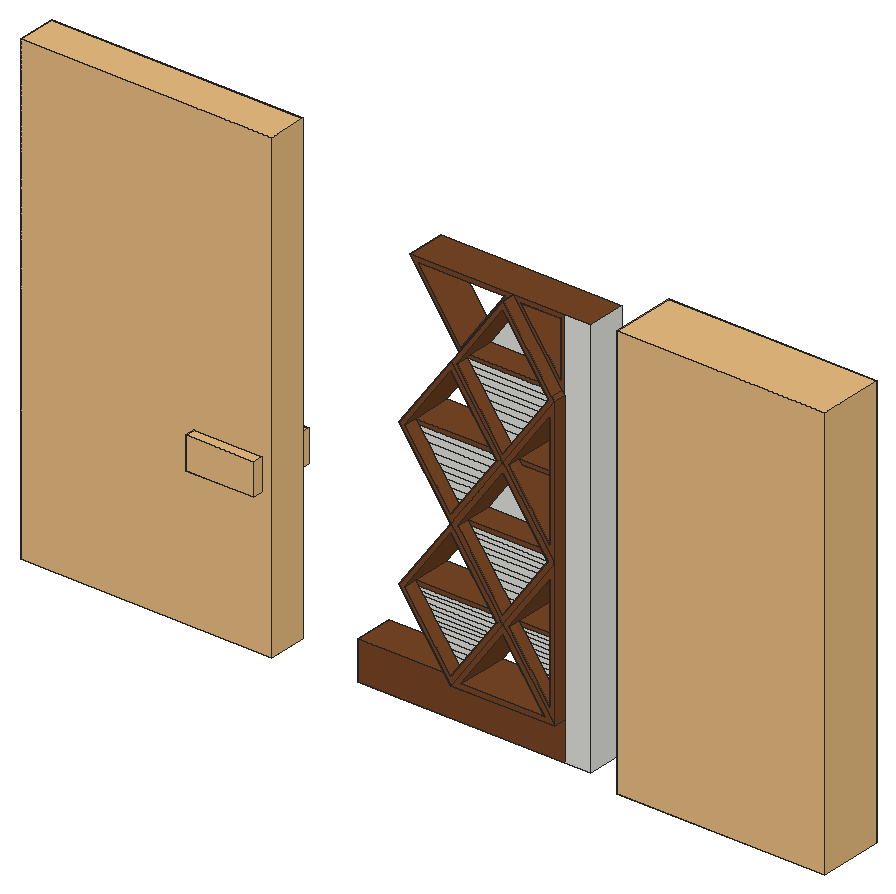
# SketchUp Ruby script. Lengths in inches.
U = 1.inch
M = Sketchup.active_model
def pt(a) = Geom::Point3d.new(a.map { |v| v * U })
def face(e, loops, mat)
  f = e.add_face(loops[0].map { |a| pt(a) })
  loops[1..].each { |l| e.add_face(l.map { |a| pt(a) }).erase! }
  f.material = f.back_material = mat if mat
  f
end
# faces: each face lists its corners as indices into pts; further lists are holes
def faces(e, pts, list, mat = nil) = list.each { |f| face(e, (f[0].is_a?(Array) ? f : [f]).map { |l| l.map { |i| pts[i] } }, mat) }
# xy, xz, yz: faces in a plane at the given z, y or x. An outline is a flat list of corners, or four numbers for a rectangle; further outlines are holes
def ring(l) = l.size == 4 ? [[l[0], l[1]], [l[2], l[1]], [l[2], l[3]], [l[0], l[3]]] : l.each_slice(2).to_a
def flat(e, list, mat, &to3) = list.each { |f| face(e, (f[0].is_a?(Array) ? f : [f]).map { |l| ring(l).map { |u, v| to3.(u, v) } }, mat) }
def xy(e, z, list, mat = nil) = flat(e, list, mat) { |x, y| [x, y, z] }
def xz(e, y, list, mat = nil) = flat(e, list, mat) { |x, z| [x, y, z] }
def yz(e, x, list, mat = nil) = flat(e, list, mat) { |y, z| [x, y, z] }
def lines(e, pts, list) = list.each { |a, b| e.add_line(pt(pts[a]), pt(pts[b])) }
# prism: a flat outline (further loops are holes) pulled along v
def prism(e, loops, v, mat = nil)
  f = face(e, loops, mat); d = Geom::Vector3d.new(v.map { |x| x * U })
  f.pushpull(f.normal.samedirection?(d) ? d.length : -d.length)
end
def box(e, o, s, mat = nil) = prism(e, [[o, [o[0] + s[0], o[1], o[2]], [o[0] + s[0], o[1] + s[1], o[2]], [o[0], o[1] + s[1], o[2]]]], [0, 0, s[2]], mat)
def at(x, y, z, deg = 0) = Geom::Transformation.translation(pt([x, y, z])) * Geom::Transformation.rotation(ORIGIN, Z_AXIS, deg.degrees)
def axes(o, x, y, z) = Geom::Transformation.new([*x, 0, *y, 0, *z, 0, *pt(o).to_a, 1])
def part(name) = M.definitions.add(name)
# library, detail: a bought-in or finely detailed component or shape, given as its bounding box
def library(name, o, s) = part(name).tap { |d| box(d.entities, o, s) }
def detail(e, o, s) = box(e.add_group.entities, o, s)
def put(e, d, t, mat = nil) = e.add_instance(d, t).tap { |i| i.material = mat if mat }
def group(e, t, mat = nil) = e.add_group.tap { |g| g.transformation = t; g.material = mat if mat }.entities
root = M.entities
M.materials.add("[Wood Veneer 01]").color = [120, 70, 37]
c1 = library("Group4\#1",[-223.39,66.61,0],[17.37,17.18,34.03])
c2 = library("Group145\#1",[5.875,6.46,9.56],[20.8,10.13,11.36])
c3 = library("Redhome_Model_Tree_04",[-24.25,-16.26,0],[46.77,28.59,38.54])
c4 = library("Deer Decoration @ADS 031224",[-97.53,29.72,25.79],[8.17,5.75,13.32])
c5 = library("MC-5",[1.46,3.91,28.72],[9.58,10.53,13.64])
c6 = library("DECOR4",[0,0,0],[6.14,2.35,8.66])
c7 = library("Vaso+com+Suculentas+e+Livro+Chanel+-+Marilia+Zimmermann",[189.86,96.28,0],[20.19,20.19,9.48])
c8 = library("Decor 1 - asm",[600.96,98.01,0],[8.71,8.72,11.09])
c9 = library("Group\#1",[0,0,0],[19.39,3,36])
c10 = library("Group43\#1",[-4.22,-4.32,0],[4.42,4.42,11.16])
c11 = library("Group43",[-4.22,-4.32,0],[4.42,4.42,11.16])
c12 = library("Group\#127",[-0.03,-0.72,0],[16.04,5,32])
xy(root,0,[[0,1,18,4]])
xy(root,2.96,[[8,0,16,1],[0,1,8,4]],"[Wood Veneer 01]")
xy(root,3.35,[[8.77,0,15.23,4]],"[Wood Veneer 01]")
xy(root,8.5625,[[4.47,1,11.53,4],[12.47,1,15.62,4]],"[Wood Veneer 01]")
xy(root,14.17,[[8.5,1,15.5,3]],"[Wood Veneer 01]")
xy(root,19.47,[[12.68,1,15.625,3]],"[Wood Veneer 01]")
xy(root,19.77,[[4.47,1,11.53,4],[12.46,1,15.625,4]],"[Wood Veneer 01]")
xy(root,25.66,[[8.66,1,15.34,3]],"[Wood Veneer 01]")
xy(root,30.66,[[4.62,1,11.38,4],[12.62,1,15.68,4]],"[Wood Veneer 01]")
xy(root,30.98,[[4,1,18,4]],"[Wood Veneer 01]")
xz(root,0,[[8,2.96,11.8,8.28,12,8.5625,11.53,8.5625,11.33,8.28,8,3.62,4.47,8.5625,8,13.5,11.53,8.5625,12,8.5625,8.24,13.83,8,14.17,4,8.5625],[[8,2.96,16,2.96,12.21,8.26,12,8.5625,11.8,8.28],[8.77,3.35,12,7.88,15.23,3.35]],[[16,2.96,16,14.17,15.76,13.83,12,8.5625,12.21,8.26],[15.62,4.14,12.68,8.26,12.47,8.5625,15.62,12.98]],[[12,8.5625,15.76,13.83,16,14.17,12,19.77,11.74,19.41,8,14.17,8.24,13.83],[12,9.26,8.74,13.83,8.5,14.17,12,19.07,15.5,14.17,15.26,13.83]],[8,14.17,11.74,19.41,12,19.77,11.53,19.77,11.27,19.41,8,14.83,4.47,19.77,8,24.72,11.53,19.77,12,19.77,8,25.375,4,19.77],
  [[16,14.17,16,25.375,12,19.77],[15.625,15.34,12.68,19.47,12.46,19.77,15.625,24.2]],[[12,19.77,16,25.375,15.8,25.66,12,30.98,8.2,25.66,8,25.375],[12,20.42,8.46,25.375,8.66,25.66,12,30.33,15.34,25.66,15.54,25.375]]],"[Wood Veneer 01]")
xz(root,1,[[16,0,18,30.98],[8,3.62,8.53,4.37,7.47,4.37],[15.62,4.14,15.62,4.99,15.02,4.99],[7.47,4.37,8.53,4.37,8.82,4.77,7.18,4.77],[7.18,4.77,8.82,4.77,9.125,5.2,6.875,5.2],
  [15.02,4.99,15.62,4.99,15.62,5.3125,14.79,5.3125],[6.875,5.2,9.125,5.2,9.45,5.65,6.55,5.65],[14.79,5.3125,15.62,5.3125,15.62,5.625,14.5625,5.625],[14.5625,5.625,15.62,5.625,15.62,5.98,14.31,5.98],[6.55,5.65,9.45,5.65,9.72,6.02,6.28,6.02],
  [14.31,5.98,15.62,5.98,15.62,6.32,14.07,6.32],[6.28,6.02,9.72,6.02,9.94,6.34,6.06,6.34],[14.07,6.32,15.62,6.32,15.62,6.68,13.81,6.68],[6.06,6.34,9.94,6.34,10.18,6.68,5.82,6.68],[5.82,6.68,10.18,6.68,10.39,6.96,5.61,6.96],
  [13.81,6.68,15.62,6.68,15.62,7.02,13.57,7.02],[5.61,6.96,10.39,6.96,10.64,7.32,5.36,7.32],[13.57,7.02,15.62,7.02,15.62,7.34,13.34,7.34],[5.36,7.32,10.64,7.32,10.9,7.68,5.1,7.68],[13.34,7.34,15.62,7.34,15.62,7.68,13.1,7.68],
  [5.1,7.68,10.9,7.68,11.125,8,4.875,8],[13.1,7.68,15.62,7.68,15.62,8.02,12.85,8.02],[4.875,8,11.125,8,11.33,8.28,4.67,8.28],[12.85,8.02,15.62,8.02,15.62,8.26,12.68,8.26],[12,9.26,12.42,9.84,11.58,9.84],
  [11.58,9.84,12.42,9.84,12.83,10.42,11.17,10.42],[11.17,10.42,12.83,10.42,13.18,10.92,10.82,10.92],[10.82,10.92,13.18,10.92,13.56,11.44,10.44,11.44],[10.44,11.44,13.56,11.44,13.85,11.85,10.15,11.85],[10.15,11.85,13.85,11.85,14.1875,12.32,9.8125,12.32],
  [9.8125,12.32,14.1875,12.32,14.48,12.74,9.52,12.74],[9.52,12.74,14.48,12.74,14.77,13.14,9.23,13.14],[9.23,13.14,14.77,13.14,15.03,13.5,8.97,13.5],[8.97,13.5,15.03,13.5,15.26,13.83,8.74,13.83],[8,14.83,8.4,15.38,7.6,15.38],
  [7.6,15.38,8.4,15.38,8.79,15.9375,7.21,15.9375],[7.21,15.9375,8.79,15.9375,9.16,16.45,6.84,16.45],[6.84,16.45,9.16,16.45,9.4375,16.84,6.5625,16.84],[6.5625,16.84,9.4375,16.84,9.79,17.33,6.21,17.33],[6.21,17.33,9.79,17.33,10.18,17.88,5.82,17.88],
  [5.82,17.88,10.18,17.88,10.58,18.45,5.42,18.45],[5.42,18.45,10.58,18.45,10.98,19,5.02,19],[5.02,19,10.98,19,11.27,19.41,4.73,19.41],[12,20.42,12.67,21.36,11.33,21.36],[11.33,21.36,12.67,21.36,13.09,21.9375,10.91,21.9375],
  [10.91,21.9375,13.09,21.9375,13.5,22.52,10.5,22.52],[10.5,22.52,13.5,22.52,13.875,23.04,10.125,23.04],[10.125,23.04,13.875,23.04,14.25,23.58,9.75,23.58],[9.75,23.58,14.25,23.58,14.54,23.98,9.46,23.98],[9.46,23.98,14.54,23.98,14.89,24.47,9.11,24.47],
  [9.11,24.47,14.89,24.47,15.21,24.91,8.79,24.91],[8.79,24.91,15.21,24.91,15.54,25.375,8.46,25.375]])
xz(root,1,[[0,0,16,2.96],[12.68,8.26,15.62,8.26,15.62,8.5625,12.47,8.5625],[4.67,8.28,11.33,8.28,11.53,8.5625,4.47,8.5625],[8.74,13.83,15.26,13.83,15.5,14.17,8.5,14.17],[4.73,19.41,11.27,19.41,11.53,19.77,4.47,19.77],
  [12.68,19.47,15.625,19.47,15.625,19.77,12.46,19.77],[[8,25.375,8.2,25.66,12,30.98,15.8,25.66,16,25.375,16,30.98,4,30.98],[8,25.92,4.62,30.66,11.38,30.66],[15.68,26.37,12.62,30.66,15.68,30.66]],[8.46,25.375,15.54,25.375,15.34,25.66,8.66,25.66]],"[Wood Veneer 01]")
xz(root,3,[[8.5,14.17,15.5,14.17,12,19.07],[8.66,25.66,15.34,25.66,12,30.33]])
xz(root,3.97,[[11.9,8.41,7.9,14.02,8,14.17,11.9,19.62,15.9,14.02]])
yz(root,0,[[1,0,4,2.96]],"[Wood Veneer 01]")
yz(root,15.62,[[0,4.14,0,12.98,4,12.98,4,8.5625,1,8.5625,1,4.14]],"[Wood Veneer 01]")
yz(root,15.625,[[0,15.34,3,19.47],[0,19.47,1,19.77],[0,19.77,4,24.2]],"[Wood Veneer 01]")
yz(root,15.68,[[1,26.37,4,30.66]],"[Wood Veneer 01]")
yz(root,16,[[0,2.96,1,25.375]],"[Wood Veneer 01]")
yz(root,18,[[1,0,4,30.98]])
p = [[4,0,8.5625],[4,4,8.5625],[8,4,2.96],[8,1,2.96],[8,0,2.96],[12,4,7.88],
  [12,0,7.88],[8.77,0,3.35],[8.77,4,3.35],[15.23,4,3.35],[15.23,0,3.35],[4.875,1,8],
  [4.67,1,8.28],[4.47,1,8.5625],[4.47,0,8.5625],[8,0,3.62],[8,1,3.62],[7.47,1,4.37],
  [7.18,1,4.77],[6.875,1,5.2],[6.55,1,5.65],[6.28,1,6.02],[6.06,1,6.34],[5.82,1,6.68],
  [5.61,1,6.96],[5.36,1,7.32],[5.1,1,7.68],[11.53,1,8.5625],[11.33,1,8.28],[11.125,1,8],
  [10.9,1,7.68],[10.64,1,7.32],[10.39,1,6.96],[10.18,1,6.68],[9.94,1,6.34],[9.72,1,6.02],
  [9.45,1,5.65],[9.125,1,5.2],[8.82,1,4.77],[8.53,1,4.37],[11.33,0,8.28],[11.53,0,8.5625],
  [12.85,1,8.02],[12.68,1,8.26],[12.47,1,8.5625],[12.47,0,8.5625],[12.68,0,8.26],[15.62,0,4.14],
  [15.62,1,4.14],[15.02,1,4.99],[14.79,1,5.3125],[14.5625,1,5.625],[14.31,1,5.98],[14.07,1,6.32],
  [13.81,1,6.68],[13.57,1,7.02],[13.34,1,7.34],[13.1,1,7.68],[11.9,1.97,8.41],[7.9,1.97,14.02],
  [7.9,3.97,14.02],[11.9,3.97,8.41],[15.9,1.97,14.02],[15.9,3.97,14.02],[8,0,14.17],[8,1.97,14.17],
  [8,3.97,14.17],[8,4,14.17],[8,4,13.5],[8,0,13.5],[4.47,4,8.5625],[11.53,4,8.5625],
  [15.62,4,12.98],[15.62,0,12.98],[12.47,4,8.5625],[8.5,0,14.17],[8.74,0,13.83],[12,0,9.26],
  [12,1,9.26],[11.58,1,9.84],[11.17,1,10.42],[10.82,1,10.92],[10.44,1,11.44],[10.15,1,11.85],
  [9.8125,1,12.32],[9.52,1,12.74],[9.23,1,13.14],[8.97,1,13.5],[8.74,1,13.83],[8.5,1,14.17],
  [15.5,1,14.17],[15.26,1,13.83],[15.03,1,13.5],[14.77,1,13.14],[14.48,1,12.74],[14.1875,1,12.32],
  [13.85,1,11.85],[13.56,1,11.44],[13.18,1,10.92],[12.83,1,10.42],[12.42,1,9.84],[15.26,0,13.83],
  [15.5,0,14.17],[11.9,1.97,19.62],[11.9,3.97,19.62],[4,0,19.77],[4,4,19.77],[12,3,19.07],
  [12,0,19.07],[8.5,3,14.17],[15.5,3,14.17],[5.02,1,19],[4.73,1,19.41],[4.47,1,19.77],
  [4.47,0,19.77],[8,0,14.83],[8,1,14.83],[7.6,1,15.38],[7.21,1,15.9375],[6.84,1,16.45],
  [6.5625,1,16.84],[6.21,1,17.33],[5.82,1,17.88],[5.42,1,18.45],[11.53,1,19.77],[11.27,1,19.41],
  [10.98,1,19],[10.58,1,18.45],[10.18,1,17.88],[9.79,1,17.33],[9.4375,1,16.84],[9.16,1,16.45],
  [8.79,1,15.9375],[8.4,1,15.38],[11.27,0,19.41],[11.53,0,19.77],[12.68,3,19.47],[12.68,1,19.47],
  [12.46,1,19.77],[12.46,0,19.77],[12.68,0,19.47],[15.625,0,15.34],[15.625,3,15.34],[8,0,25.375],
  [8,1,25.375],[8,4,25.375],[8,4,24.72],[8,0,24.72],[4.47,4,19.77],[11.53,4,19.77],
  [15.625,4,24.2],[15.625,0,24.2],[12.46,4,19.77],[8.79,1,24.91],[8.46,1,25.375],[8.46,0,25.375],
  [12,0,20.42],[12,1,20.42],[11.33,1,21.36],[10.91,1,21.9375],[10.5,1,22.52],[10.125,1,23.04],
  [9.75,1,23.58],[9.46,1,23.98],[9.11,1,24.47],[12.67,1,21.36],[15.54,0,25.375],[15.54,1,25.375],
  [15.21,1,24.91],[14.89,1,24.47],[14.54,1,23.98],[14.25,1,23.58],[13.875,1,23.04],[13.5,1,22.52],
  [13.09,1,21.9375],[12,1,30.98],[8.2,1,25.66],[8.2,0,25.66],[12,0,30.98],[8.66,1,25.66],
  [8.66,3,25.66],[12,3,30.33],[12,0,30.33],[8.66,0,25.66],[15.34,3,25.66],[15.34,1,25.66],
  [15.34,0,25.66],[16,1,25.375],[15.8,1,25.66],[15.8,0,25.66],[16,0,25.375],[4,1,30.98],
  [4,4,30.98],[4.62,1,30.66],[8,1,25.92],[8,4,25.92],[4.62,4,30.66],[11.38,1,30.66],
  [11.38,4,30.66],[12.62,1,30.66],[15.68,1,26.37],[15.68,4,26.37],[12.62,4,30.66],[15.62,1,8.5625],
  [15.625,1,8.5625],[11.74,1,19.41],[11.74,0,19.41],[15.76,1,13.83],[15.76,0,13.83],[8.24,1,13.83],
  [8.24,0,13.83],[12.21,1,8.26],[12.21,0,8.26],[14.8125,1,12.32]]
faces(root,p,[[0,1,2,3,4],[5,6,7,8],[9,10,6,5],[11,12,13,14,15,16,17,18,19,20,21,22,23,24,25,26],[27,28,29,30,31,32,33,34,35,36,37,38,39,16,15,40,41],[42,43,44,45,46,47,48,49,50,51,52,53,54,55,56,57],[64,65,59,60,66,67,1,0],[68,69,14,13,70],
  [71,27,41,69,68],[72,73,45,44,74],[75,76,77,78,79,80,81,82,83,84,85,86,87,88,89],[90,91,92,93,94,95,96,97,98,99,100,78,77,101,102],[59,65,66,60],[67,66,65,64,105,106],[107,108,75,89,109],[110,90,102,108,107],
  [111,112,113,114,115,116,117,118,119,120,121,122,123],[124,125,126,127,128,129,130,131,132,133,116,115,134,135],[136,137,138,139,140,141,142],[143,144,145,106,105],[146,147,114,113,148],[149,124,135,147,146],[150,151,139,138,152],[153,154,155,156,157,158,159,160,161,162,163,164],
  [165,157,156,166,167,168,169,170,171,172,173,174],[175,176,144,143,177,178],[154,179,180,181,182,183,155],[184,185,167,166,186,182,181],[187,188,189,190],[144,191,192,145],[188,175,178,189],[193,194,195,196],
  [194,197,198,195],[199,200,201,202]],"[Wood Veneer 01]")
faces(root,p,[[58,59,60,61],[62,58,61,63],[103,62,63,104],[104,66,65,103]])
lines(root,p,[[203,204],[205,206],[207,208],[209,210],[211,212],[95,213]])
put(root,c1,axes([14.24,-8.97,1.96],[0.1386,0,0],[0,0.1386,0],[0,0,0.1386]))
put(root,c2,axes([-17.72,-0.25,17.05],[0.17037,0,0],[0,0.12267,0],[0,0,0.31282]))
put(root,c3,axes([-9.42,1.67,28.91],[0.0792,0,0],[0,0.0792,0],[0,0,0.0792]))
put(root,c4,axes([21.27,-11.04,-1.8],[0.39,0,0],[0,0.39,0],[0,0,0.39]))
put(root,c5,axes([-14.13,-0.3125,9.1],[0.11622,0.13136,0],[-0.13136,0.11622,0],[0,0,0.17539]))
put(root,c6,axes([-10.76,0.91,17.1],[0.3773,0,0],[0,0.3773,0],[0,0,0.3773]))
put(root,c7,axes([-61.24,-25.77,11.1875],[0.26,0,0],[0,0.26,0],[0,0,0.26]))
put(root,c8,axes([-119.81,-15.1,5.22],[0.16509,0,0],[0,0.16509,0],[0,0,0.16509]))
put(root,c9,at(-25.29,0.03,0))
put(root,c10,axes([-9.93,2.42,5.29],[0.2397,0,0],[0,0.2397,0],[0,0,0.2397]))
put(root,c11,axes([-7.97,2.79,5.29],[0.32563,0,0],[0,0.32563,0],[0,0,0.32563]))
put(root,c12,at(20.85,0.72,0))
